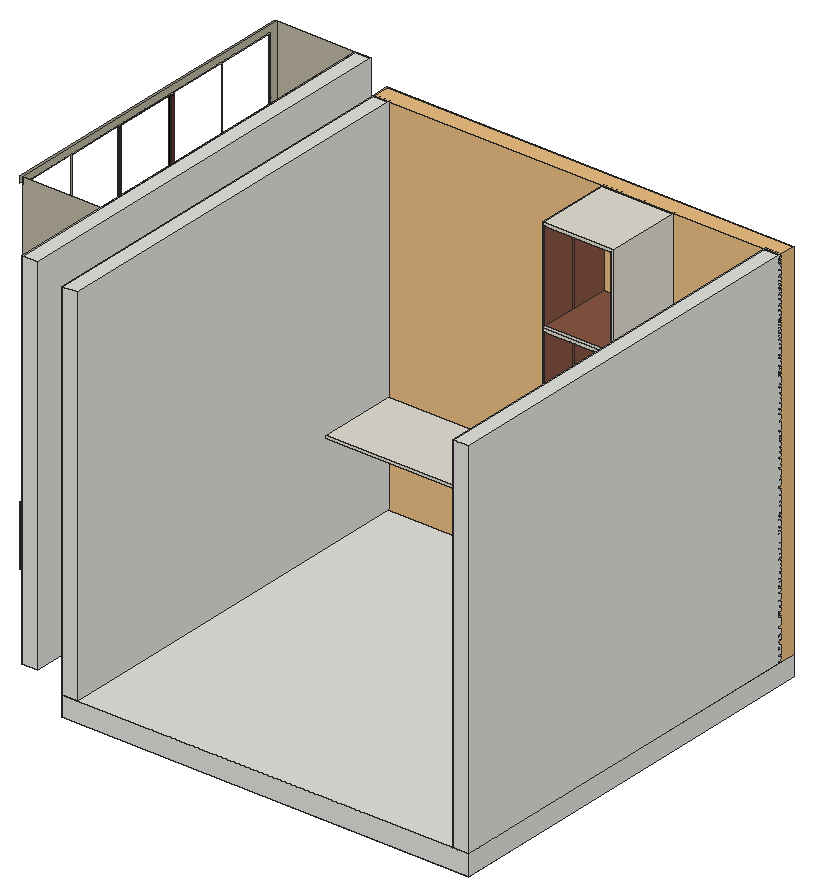
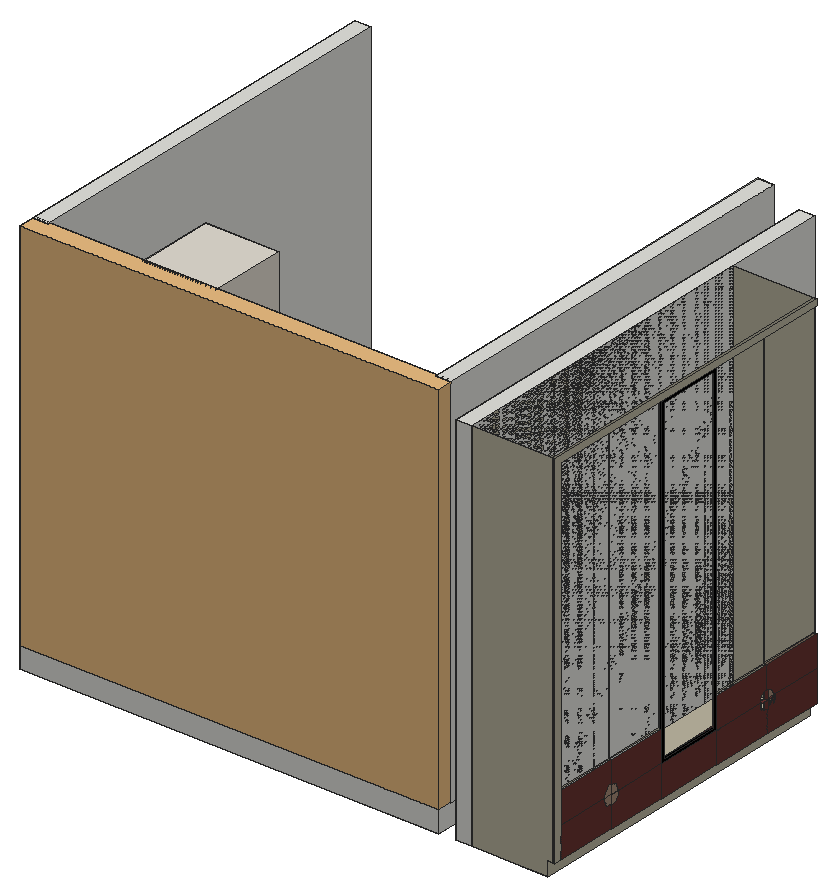
# SketchUp Ruby script. Lengths in millimetres.
U = 1.mm
M = Sketchup.active_model
def pt(a) = Geom::Point3d.new(a.map { |v| v * U })
def face(e, loops, mat)
  f = e.add_face(loops[0].map { |a| pt(a) })
  loops[1..].each { |l| e.add_face(l.map { |a| pt(a) }).erase! }
  f.material = f.back_material = mat if mat
  f
end
# faces: each face lists its corners as indices into pts; further lists are holes
def faces(e, pts, list, mat = nil) = list.each { |f| face(e, (f[0].is_a?(Array) ? f : [f]).map { |l| l.map { |i| pts[i] } }, mat) }
# xy, xz, yz: faces in a plane at the given z, y or x. An outline is a flat list of corners, or four numbers for a rectangle; further outlines are holes
def ring(l) = l.size == 4 ? [[l[0], l[1]], [l[2], l[1]], [l[2], l[3]], [l[0], l[3]]] : l.each_slice(2).to_a
def flat(e, list, mat, &to3) = list.each { |f| face(e, (f[0].is_a?(Array) ? f : [f]).map { |l| ring(l).map { |u, v| to3.(u, v) } }, mat) }
def xy(e, z, list, mat = nil) = flat(e, list, mat) { |x, y| [x, y, z] }
def xz(e, y, list, mat = nil) = flat(e, list, mat) { |x, z| [x, y, z] }
def yz(e, x, list, mat = nil) = flat(e, list, mat) { |y, z| [x, y, z] }
def lines(e, pts, list) = list.each { |a, b| e.add_line(pt(pts[a]), pt(pts[b])) }
# prism: a flat outline (further loops are holes) pulled along v
def prism(e, loops, v, mat = nil)
  f = face(e, loops, mat); d = Geom::Vector3d.new(v.map { |x| x * U })
  f.pushpull(f.normal.samedirection?(d) ? d.length : -d.length)
end
def box(e, o, s, mat = nil) = prism(e, [[o, [o[0] + s[0], o[1], o[2]], [o[0] + s[0], o[1] + s[1], o[2]], [o[0], o[1] + s[1], o[2]]]], [0, 0, s[2]], mat)
def at(x, y, z, deg = 0) = Geom::Transformation.translation(pt([x, y, z])) * Geom::Transformation.rotation(ORIGIN, Z_AXIS, deg.degrees)
def axes(o, x, y, z) = Geom::Transformation.new([*x, 0, *y, 0, *z, 0, *pt(o).to_a, 1])
def part(name) = M.definitions.add(name)
# library, detail: a bought-in or finely detailed component or shape, given as its bounding box
def library(name, o, s) = part(name).tap { |d| box(d.entities, o, s) }
def detail(e, o, s) = box(e.add_group.entities, o, s)
def put(e, d, t, mat = nil) = e.add_instance(d, t).tap { |i| i.material = mat if mat }
def group(e, t, mat = nil) = e.add_group.tap { |g| g.transformation = t; g.material = mat if mat }.entities
root = M.entities
M.materials.add("Olon-Fresh-Linen-VT10-1K").color = [226, 220, 209]
M.materials.add("Pionite-a-Panolam-Brand-Canyon-Shadow-SO200-4K").color = [135, 86, 67]
M.materials.add("Tafisa-Chateau-de-Sable-or-Sand-Castle-PM782-2K").color = [163, 138, 119]
M.materials.add("Uniboard-L17-Ambrette-4K").color = [104, 52, 49]
M.materials.add("Uniboard-L19-Putty-4K").color = [187, 181, 160]
M.materials.add("[Color M09]").color = [0, 0, 0]
c1 = library("Group\#21",[0,-18,0],[3048,132.3,2743.2])
c2 = part("Group282\#1")
p = [[0,0,0],[0,0,-404.7],[-1.4,0,-404.7],[9,-1301.3,0],[-9,-1301.3,0],[9,1301.3,0],
  [9,0,0],[-9,1301.3,0],[1.4,0,-404.7],[-9,0,0],[0,0,-655.2]]
lines(c2.entities,p,[[0,1],[1,2],[3,4],[5,6],[7,5],[1,8],[9,0],[0,6],[8,10],[4,9],[6,3],[2,10],
  [9,7]])
c3 = part("Rectangle Light\#2")
put(c3.entities,c2,at(0,0,0))
c4 = library("Group\#30",[0,0,0],[533.4,18,720.8])
c5 = part("Group280\#1")
p = [[0,0,0],[0,0,-404.7],[-1.4,0,-404.7],[9,-1301.3,0],[-9,-1301.3,0],[9,1301.3,0],
  [9,0,0],[-9,1301.3,0],[1.4,0,-404.7],[-9,0,0],[0,0,-655.2]]
lines(c5.entities,p,[[0,1],[1,2],[3,4],[5,6],[7,5],[1,8],[9,0],[0,6],[8,10],[4,9],[6,3],[2,10],
  [9,7]])
c6 = part("Rectangle Light\#1")
put(c6.entities,c5,at(0,0,0))
xy(root,152.4,[[2679.7,879.2,3238.5,3258.8]],"Uniboard-L19-Putty-4K")
xy(root,254,[[2628.9,879.2,2646.9,1333.4]],"Tafisa-Chateau-de-Sable-or-Sand-Castle-PM782-2K")
xy(root,254,[[2646.9,879.2,2646.9,1336.4,2628.9,1336.4,2628.9,1790.6,2646.9,1790.6,2646.9,1793.6,2628.9,1793.6,2628.9,2290.6,2646.9,2290.6,2646.9,2293.6,2628.9,2293.6,2628.9,2747.8,2646.9,2747.8,2646.9,2750.8,2628.9,2750.8,2628.9,3205,2646.9,3205,2646.9,3208,2679.7,3208,2679.7,879.2]],"Uniboard-L17-Ambrette-4K")
xy(root,254,[[2628.9,3208,2646.9,3258.8],[2646.9,3208,2679.7,3258.8]],"Uniboard-L19-Putty-4K")
xy(root,413.1,[[2628.9,1332.9,2646.9,1333.4]],"Tafisa-Chateau-de-Sable-or-Sand-Castle-PM782-2K")
xy(root,478.1,[[2628.9,879.2,2646.9,1269.9],[2619.9,1269.9,2646.9,1333.4],[2619.9,1336.4,2646.9,1336.4,2646.9,1790.6,2628.9,1790.6,2628.9,1399.9,2619.9,1399.9],[2628.9,1793.6,2646.9,2290.6],[2628.9,2293.6,2646.9,2747.8],
  [2628.9,2750.8,2646.9,3205]],"Uniboard-L17-Ambrette-4K")
xy(root,481.1,[[2628.9,879.2,2646.9,1269.9],[2619.9,1269.9,2631.9,1333.4],[2631.9,1269.9,2646.9,1333.4],[2619.9,1336.4,2619.9,1399.9,2628.9,1399.9,2628.9,1790.6,2646.9,1790.6,2646.9,1336.4],[2628.9,2293.6,2646.9,2747.8],
  [2628.9,2750.8,2646.9,3205]],"Uniboard-L17-Ambrette-4K")
xy(root,481.1,[[2628.9,1793.6,2646.9,2290.6],[2646.9,1793.6,2649.9,2290.6]],"Uniboard-L19-Putty-4K")
xz(root,879.2,[[2628.9,254,2646.9,478.1],[2628.9,481.1,2646.9,705.2]],"Uniboard-L17-Ambrette-4K")
xz(root,879.2,[[2679.7,152.4,3238.5,152.4,3238.5,2895.6,2646.9,2895.6,2646.9,254,2679.7,254]],"Uniboard-L19-Putty-4K")
xz(root,1269.9,[[2628.9,476.1,2646.9,478.1],[2628.9,481.1,2631.9,483.1],[2631.9,481.1,2646.9,483.1]],"Tafisa-Chateau-de-Sable-or-Sand-Castle-PM782-2K")
xz(root,1269.9,[[2619.9,476.1,2628.9,478.1],[2619.9,481.1,2628.9,483.1]],"Uniboard-L17-Ambrette-4K")
xz(root,1333.4,[[2628.9,254,2646.9,413.1],[2619.9,413.1,2646.9,478.1],[2619.9,481.1,2631.9,546.1],[2631.9,481.1,2646.9,546.1]],"Uniboard-L17-Ambrette-4K")
xz(root,1336.4,[[2628.9,254,2646.9,254,2646.9,478.1,2619.9,478.1,2619.9,413.1,2628.9,413.1],[2619.9,481.1,2646.9,481.1,2646.9,705.2,2628.9,705.2,2628.9,546.1,2619.9,546.1]],"Uniboard-L17-Ambrette-4K")
xz(root,1399.9,[[2619.9,476.1,2628.9,478.1],[2619.9,481.1,2628.9,483.1]],"Uniboard-L17-Ambrette-4K")
xz(root,1790.6,[[2628.9,254,2646.9,478.1],[2628.9,481.1,2646.9,705.2]],"Uniboard-L17-Ambrette-4K")
xz(root,1793.6,[[2628.9,254,2646.9,478.1]],"Uniboard-L17-Ambrette-4K")
xz(root,1793.6,[[2646.9,481.1,2649.9,2841.8]],"Uniboard-L19-Putty-4K")
xz(root,1793.6,[[2628.9,481.1,2646.9,2841.8]],"[Color M09]")
xz(root,2290.6,[[2628.9,254,2646.9,478.1]],"Uniboard-L17-Ambrette-4K")
xz(root,2290.6,[[2646.9,481.1,2649.9,2841.8]],"Uniboard-L19-Putty-4K")
xz(root,2290.6,[[2628.9,481.1,2646.9,2841.8]],"[Color M09]")
xz(root,2293.6,[[2628.9,254,2646.9,478.1],[2628.9,481.1,2646.9,705.2]],"Uniboard-L17-Ambrette-4K")
xz(root,2747.8,[[2628.9,254,2646.9,478.1],[2628.9,481.1,2646.9,705.2]],"Uniboard-L17-Ambrette-4K")
xz(root,2750.8,[[2628.9,254,2646.9,478.1],[2628.9,481.1,2646.9,705.2]],"Uniboard-L17-Ambrette-4K")
xz(root,3205,[[2628.9,254,2646.9,478.1]],"Tafisa-Chateau-de-Sable-or-Sand-Castle-PM782-2K")
xz(root,3205,[[2628.9,481.1,2646.9,705.2]],"Uniboard-L17-Ambrette-4K")
xz(root,3208,[[2628.9,254,2646.9,2844.8]],"Uniboard-L19-Putty-4K")
xz(root,3258.8,[[2679.7,152.4,2679.7,254,2646.9,254,2646.9,2895.6,3238.5,2895.6,3238.5,152.4],[2628.9,254,2646.9,2895.6]],"Uniboard-L19-Putty-4K")
yz(root,2628.9,[[2747.3,413.1,2747.8,413.1,2747.8,478.1,2684.3,478.1,2684.3,476.1,2684.4,474,2684.8,470,2685.1,467.9,2686.3,461.9,2686.9,460,2687.5,458,2688.1,456.1,2690.5,450.4,2692.3,446.8,2693.4,445,2694.4,443.3,2695.5,441.6,2696.7,439.9,2697.9,438.3,2700.5,435.1,2703.3,432.1,2706.3,429.3,2709.5,426.7,2711.1,425.5,2712.8,424.3,2714.5,423.2,2716.2,422.2,2718,421.1,2721.6,419.3,2723.5,418.4,2725.4,417.7,2727.3,416.9,2729.2,416.3,2731.2,415.7,2733.1,415.1,2739.1,413.9,2741.2,413.6,2745.2,413.2],[2750.8,413.1,2751.3,413.1,2753.4,413.2,2755.4,413.4,2757.5,413.6,2759.5,413.9,2765.5,415.1,2767.4,415.7,2769.4,416.3,2771.3,416.9,2773.2,417.7,2775.1,418.4,2777,419.3,2780.6,421.1,2782.4,422.2,2784.1,423.2,2785.8,424.3,2787.5,425.5,2789.1,426.7,2792.3,429.3,2795.3,432.1,2798.1,435.1,2800.7,438.3,2801.9,439.9,2803.1,441.6,2805.3,445,2806.3,446.8,2808.1,450.4,2809,452.3,2809.7,454.2,2810.5,456.1,2811.1,458,2811.7,460,2812.3,461.9,2812.7,463.9,2813.2,465.9,2813.5,467.9,2813.8,470,2814.2,474,2814.3,476.1,2814.3,478.1,2750.8,478.1],[2684.3,481.1,2747.8,481.1,2747.8,546.1,2747.3,546.1,2745.2,546,2741.2,545.6,2739.1,545.3,2733.1,544.1,2731.2,543.5,2729.2,542.9,2727.3,542.3,2725.4,541.5,2723.5,540.8,2721.6,539.9,2718,538.1,2716.2,537,2714.5,536,2712.8,534.9,2711.1,533.7,2709.5,532.5,2706.3,529.9,2703.3,527.1,2700.5,524.1,2697.9,520.9,2696.7,519.3,2695.5,517.6,2694.4,515.9,2693.4,514.2,2692.3,512.4,2690.5,508.8,2688.1,503.1,2687.5,501.2,2686.9,499.2,2686.3,497.3,2685.1,491.3,2684.8,489.2,2684.4,485.2,2684.3,483.1],[2750.8,481.1,2814.3,481.1,2814.3,483.1,2814.2,485.2,2813.8,489.2,2813.5,491.3,2813.2,493.3,2812.7,495.3,2812.3,497.3,2811.7,499.2,2811.1,501.2,2810.5,503.1,2809.7,505,2809,506.9,2808.1,508.8,2806.3,512.4,2805.3,514.2,2803.1,517.6,2801.9,519.3,2800.7,520.9,2798.1,524.1,2795.3,527.1,2792.3,529.9,2789.1,532.5,2787.5,533.7,2785.8,534.9,2784.1,536,2782.4,537,2780.6,538.1,2777,539.9,2775.1,540.8,2773.2,541.5,2771.3,542.3,2769.4,542.9,2767.4,543.5,2765.5,544.1,2759.5,545.3,2757.5,545.6,2755.4,545.8,2753.4,546,2751.3,546.1,2750.8,546.1]],"Tafisa-Chateau-de-Sable-or-Sand-Castle-PM782-2K")
yz(root,2628.9,[[879.2,254,879.2,478.1,1269.9,478.1,1269.9,476.1,1270,474,1270.4,470,1270.7,467.9,1271.9,461.9,1272.5,460,1273.1,458,1273.7,456.1,1276.1,450.4,1277.9,446.8,1279,445,1280,443.3,1281.1,441.6,1282.3,439.9,1283.5,438.3,1286.1,435.1,1288.9,432.1,1291.9,429.3,1295.1,426.7,1296.7,425.5,1298.4,424.3,1300.1,423.2,1301.8,422.2,1303.6,421.1,1307.2,419.3,1309.1,418.4,1311,417.7,1312.9,416.9,1314.8,416.3,1316.8,415.7,1318.7,415.1,1324.7,413.9,1326.8,413.6,1330.8,413.2,1332.9,413.1,1333.4,413.1,1333.4,254],[1336.4,254,1336.4,413.1,1336.9,413.1,1339,413.2,1341,413.4,1343.1,413.6,1345.1,413.9,1351.1,415.1,1353,415.7,1355,416.3,1356.9,416.9,1358.8,417.7,1360.7,418.4,1362.6,419.3,1366.2,421.1,1368,422.2,1369.7,423.2,1371.4,424.3,1373.1,425.5,1374.7,426.7,1377.9,429.3,1380.9,432.1,1383.7,435.1,1386.3,438.3,1387.5,439.9,1388.7,441.6,1390.9,445,1391.9,446.8,1393.7,450.4,1394.6,452.3,1395.3,454.2,1396.1,456.1,1396.7,458,1397.3,460,1397.9,461.9,1398.3,463.9,1398.8,465.9,1399.1,467.9,1399.4,470,1399.8,474,1399.9,476.1,1399.9,478.1,1790.6,478.1,1790.6,254],[1793.6,254,2290.6,478.1],[2293.6,254,2293.6,478.1,2684.3,478.1,2684.3,476.1,2684.4,474,2684.8,470,2685.1,467.9,2686.3,461.9,2686.9,460,2687.5,458,2688.1,456.1,2690.5,450.4,2692.3,446.8,2693.4,445,2694.4,443.3,2695.5,441.6,2696.7,439.9,2697.9,438.3,2700.5,435.1,2703.3,432.1,2706.3,429.3,2709.5,426.7,2711.1,425.5,2712.8,424.3,2714.5,423.2,2716.2,422.2,2718,421.1,2721.6,419.3,2723.5,418.4,2725.4,417.7,2727.3,416.9,2729.2,416.3,2731.2,415.7,2733.1,415.1,2739.1,413.9,2741.2,413.6,2745.2,413.2,2747.3,413.1,2747.8,413.1,2747.8,254],[2750.8,254,2750.8,413.1,2751.3,413.1,2753.4,413.2,2755.4,413.4,2757.5,413.6,2759.5,413.9,2765.5,415.1,2767.4,415.7,2769.4,416.3,2771.3,416.9,2773.2,417.7,2775.1,418.4,2777,419.3,2780.6,421.1,2782.4,422.2,2784.1,423.2,2785.8,424.3,2787.5,425.5,2789.1,426.7,2792.3,429.3,2795.3,432.1,2798.1,435.1,2800.7,438.3,2801.9,439.9,2803.1,441.6,2805.3,445,2806.3,446.8,2808.1,450.4,2809,452.3,2809.7,454.2,2810.5,456.1,2811.1,458,2811.7,460,2812.3,461.9,2812.7,463.9,2813.2,465.9,2813.5,467.9,2813.8,470,2814.2,474,2814.3,476.1,2814.3,478.1,3205,478.1,3205,254],
  [879.2,481.1,879.2,705.2,1333.4,705.2,1333.4,546.1,1332.9,546.1,1330.8,546,1326.8,545.6,1324.7,545.3,1318.7,544.1,1316.8,543.5,1314.8,542.9,1312.9,542.3,1311,541.5,1309.1,540.8,1307.2,539.9,1303.6,538.1,1301.8,537,1300.1,536,1298.4,534.9,1296.7,533.7,1295.1,532.5,1291.9,529.9,1288.9,527.1,1286.1,524.1,1283.5,520.9,1282.3,519.3,1281.1,517.6,1280,515.9,1279,514.2,1277.9,512.4,1276.1,508.8,1273.7,503.1,1273.1,501.2,1272.5,499.2,1271.9,497.3,1270.7,491.3,1270.4,489.2,1270,485.2,1269.9,483.1,1269.9,481.1],[1399.9,481.1,1399.9,483.1,1399.8,485.2,1399.4,489.2,1399.1,491.3,1398.8,493.3,1398.3,495.3,1397.9,497.3,1397.3,499.2,1396.7,501.2,1396.1,503.1,1395.3,505,1394.6,506.9,1393.7,508.8,1391.9,512.4,1390.9,514.2,1388.7,517.6,1387.5,519.3,1386.3,520.9,1383.7,524.1,1380.9,527.1,1377.9,529.9,1374.7,532.5,1373.1,533.7,1371.4,534.9,1369.7,536,1368,537,1366.2,538.1,1362.6,539.9,1360.7,540.8,1358.8,541.5,1356.9,542.3,1355,542.9,1353,543.5,1351.1,544.1,1345.1,545.3,1343.1,545.6,1341,545.8,1339,546,1336.9,546.1,1336.4,546.1,1336.4,705.2,1790.6,705.2,1790.6,481.1],[2293.6,481.1,2293.6,705.2,2747.8,705.2,2747.8,546.1,2747.3,546.1,2745.2,546,2741.2,545.6,2739.1,545.3,2733.1,544.1,2731.2,543.5,2729.2,542.9,2727.3,542.3,2725.4,541.5,2723.5,540.8,2721.6,539.9,2718,538.1,2716.2,537,2714.5,536,2712.8,534.9,2711.1,533.7,2709.5,532.5,2706.3,529.9,2703.3,527.1,2700.5,524.1,2697.9,520.9,2696.7,519.3,2695.5,517.6,2694.4,515.9,2693.4,514.2,2692.3,512.4,2690.5,508.8,2688.1,503.1,2687.5,501.2,2686.9,499.2,2686.3,497.3,2685.1,491.3,2684.8,489.2,2684.4,485.2,2684.3,483.1,2684.3,481.1],[2814.3,481.1,2814.3,483.1,2814.2,485.2,2813.8,489.2,2813.5,491.3,2813.2,493.3,2812.7,495.3,2812.3,497.3,2811.7,499.2,2811.1,501.2,2810.5,503.1,2809.7,505,2809,506.9,2808.1,508.8,2806.3,512.4,2805.3,514.2,2803.1,517.6,2801.9,519.3,2800.7,520.9,2798.1,524.1,2795.3,527.1,2792.3,529.9,2789.1,532.5,2787.5,533.7,2785.8,534.9,2784.1,536,2782.4,537,2780.6,538.1,2777,539.9,2775.1,540.8,2773.2,541.5,2771.3,542.3,2769.4,542.9,2767.4,543.5,2765.5,544.1,2759.5,545.3,2757.5,545.6,2755.4,545.8,2753.4,546,2751.3,546.1,2750.8,546.1,2750.8,705.2,3205,705.2,3205,481.1]],"Uniboard-L17-Ambrette-4K")
yz(root,2628.9,[[3208,254,3208,2844.8,879.2,2844.8,879.2,2895.6,3258.8,2895.6,3258.8,254]],"Uniboard-L19-Putty-4K")
yz(root,2628.9,[[[1793.6,481.1,2290.6,2841.8],[1811.6,499.1,2272.6,2823.8]]],"[Color M09]")
yz(root,2631.9,[[1269.9,481.1,1333.4,481.1,1333.4,546.1,1332.9,546.1,1330.8,546,1326.8,545.6,1324.7,545.3,1318.7,544.1,1316.8,543.5,1314.8,542.9,1312.9,542.3,1311,541.5,1309.1,540.8,1307.2,539.9,1303.6,538.1,1301.8,537,1300.1,536,1298.4,534.9,1296.7,533.7,1295.1,532.5,1291.9,529.9,1288.9,527.1,1286.1,524.1,1283.5,520.9,1282.3,519.3,1281.1,517.6,1280,515.9,1279,514.2,1277.9,512.4,1276.1,508.8,1273.7,503.1,1273.1,501.2,1272.5,499.2,1271.9,497.3,1270.7,491.3,1270.4,489.2,1270,485.2,1269.9,483.1]],"Tafisa-Chateau-de-Sable-or-Sand-Castle-PM782-2K")
yz(root,2646.9,[[879.2,254,1333.4,254,1333.4,413.1,1332.9,413.1,1330.8,413.2,1326.8,413.6,1324.7,413.9,1318.7,415.1,1316.8,415.7,1314.8,416.3,1312.9,416.9,1311,417.7,1309.1,418.4,1307.2,419.3,1303.6,421.1,1301.8,422.2,1300.1,423.2,1298.4,424.3,1296.7,425.5,1295.1,426.7,1291.9,429.3,1288.9,432.1,1286.1,435.1,1283.5,438.3,1282.3,439.9,1281.1,441.6,1280,443.3,1279,445,1277.9,446.8,1276.1,450.4,1273.7,456.1,1273.1,458,1272.5,460,1271.9,461.9,1270.7,467.9,1270.4,470,1270,474,1269.9,476.1,1269.9,478.1,879.2,478.1],[879.2,481.1,1269.9,481.1,1269.9,483.1,1270,485.2,1270.4,489.2,1270.7,491.3,1271.9,497.3,1272.5,499.2,1273.1,501.2,1273.7,503.1,1276.1,508.8,1277.9,512.4,1279,514.2,1280,515.9,1281.1,517.6,1282.3,519.3,1283.5,520.9,1286.1,524.1,1288.9,527.1,1291.9,529.9,1295.1,532.5,1296.7,533.7,1298.4,534.9,1300.1,536,1301.8,537,1303.6,538.1,1307.2,539.9,1309.1,540.8,1311,541.5,1312.9,542.3,1314.8,542.9,1316.8,543.5,1318.7,544.1,1324.7,545.3,1326.8,545.6,1330.8,546,1332.9,546.1,1333.4,546.1,1333.4,705.2,879.2,705.2]],"Tafisa-Chateau-de-Sable-or-Sand-Castle-PM782-2K")
yz(root,2646.9,[[3208,254,3258.8,254,3258.8,2895.6,879.2,2895.6,879.2,2844.8,3208,2844.8],[[1333.4,254,1333.4,478.1,879.2,478.1,879.2,481.1,1333.4,481.1,1333.4,705.2,879.2,705.2,879.2,708.2,1333.4,708.2,1333.4,2841.8,879.2,2841.8,879.2,2844.8,3208,2844.8,3208,254,3205,254,3205,478.1,2750.8,478.1,2750.8,254,2747.8,254,2747.8,478.1,2293.6,478.1,2293.6,254,2290.6,254,2290.6,478.1,1793.6,478.1,1793.6,254,1790.6,254,1790.6,478.1,1336.4,478.1,1336.4,254],[1793.6,481.1,2290.6,2841.8],[2293.6,708.2,2747.8,2841.8],[2750.8,708.2,3205,2841.8],[1336.4,708.2,1790.6,2841.8],[2293.6,481.1,2747.8,705.2],[2750.8,481.1,3205,705.2],[1336.4,481.1,1790.6,705.2]]],"Uniboard-L19-Putty-4K")
yz(root,2646.9,[[1793.6,481.1,2272.6,499.1],[2272.6,481.1,2290.6,2823.8]],"[Color M09]")
yz(root,2649.9,[[1793.6,481.1,1793.6,499.1,2272.6,499.1,2272.6,2823.8,2290.6,2823.8,2290.6,481.1]],"Uniboard-L17-Ambrette-4K")
yz(root,2679.7,[[879.2,152.4,3258.8,254]],"Uniboard-L19-Putty-4K")
yz(root,3238.5,[[879.2,152.4,3258.8,2895.6]],"Uniboard-L19-Putty-4K")
p = [[2628.9,1332.9,413.1],[2628.9,1330.8,413.2],[2646.9,1330.8,413.2],[2646.9,1332.9,413.1],[2628.9,1328.8,413.4],[2646.9,1328.8,413.4],
  [2628.9,1326.8,413.6],[2646.9,1326.8,413.6],[2628.9,1324.7,413.9],[2646.9,1324.7,413.9],[2628.9,1322.7,414.3],[2646.9,1322.7,414.3],
  [2628.9,1320.7,414.7],[2646.9,1320.7,414.7],[2628.9,1318.7,415.1],[2646.9,1318.7,415.1],[2628.9,1316.8,415.7],[2646.9,1316.8,415.7],
  [2628.9,1314.8,416.3],[2646.9,1314.8,416.3],[2628.9,1312.9,416.9],[2646.9,1312.9,416.9],[2628.9,1311,417.7],[2646.9,1311,417.7],
  [2628.9,1309.1,418.4],[2646.9,1309.1,418.4],[2628.9,1307.2,419.3],[2646.9,1307.2,419.3],[2628.9,1305.4,420.2],[2646.9,1305.4,420.2],
  [2628.9,1303.6,421.1],[2646.9,1303.6,421.1],[2628.9,1301.8,422.2],[2646.9,1301.8,422.2],[2628.9,1300.1,423.2],[2646.9,1300.1,423.2],
  [2628.9,1298.4,424.3],[2646.9,1298.4,424.3],[2628.9,1296.7,425.5],[2646.9,1296.7,425.5],[2628.9,1295.1,426.7],[2646.9,1295.1,426.7],
  [2628.9,1293.5,428],[2646.9,1293.5,428],[2628.9,1291.9,429.3],[2646.9,1291.9,429.3],[2628.9,1290.4,430.7],[2646.9,1290.4,430.7],
  [2628.9,1288.9,432.1],[2646.9,1288.9,432.1],[2628.9,1287.5,433.6],[2646.9,1287.5,433.6],[2628.9,1286.1,435.1],[2646.9,1286.1,435.1],
  [2628.9,1284.8,436.7],[2646.9,1284.8,436.7],[2628.9,1283.5,438.3],[2646.9,1283.5,438.3],[2628.9,1282.3,439.9],[2619.9,1282.3,439.9],
  [2619.9,1283.5,438.3],[2646.9,1282.3,439.9],[2628.9,1387.5,439.9],[2628.9,1386.3,438.3],[2619.9,1386.3,438.3],[2619.9,1387.5,439.9],
  [2628.9,1281.1,441.6],[2619.9,1281.1,441.6],[2646.9,1281.1,441.6],[2628.9,1388.7,441.6],[2619.9,1388.7,441.6],[2628.9,1280,443.3],
  [2619.9,1280,443.3],[2646.9,1280,443.3],[2628.9,1389.8,443.3],[2619.9,1389.8,443.3],[2628.9,1279,445],[2619.9,1279,445],
  [2646.9,1279,445],[2628.9,1390.9,445],[2619.9,1390.9,445],[2628.9,1277.9,446.8],[2619.9,1277.9,446.8],[2646.9,1277.9,446.8],
  [2628.9,1391.9,446.8],[2619.9,1391.9,446.8],[2628.9,1277,448.6],[2619.9,1277,448.6],[2646.9,1277,448.6],[2628.9,1392.8,448.6],
  [2619.9,1392.8,448.6],[2628.9,1276.1,450.4],[2619.9,1276.1,450.4],[2646.9,1276.1,450.4],[2628.9,1393.7,450.4],[2619.9,1393.7,450.4],
  [2628.9,1275.3,452.3],[2619.9,1275.3,452.3],[2646.9,1275.3,452.3],[2628.9,1394.6,452.3],[2619.9,1394.6,452.3],[2628.9,1274.5,454.2],
  [2619.9,1274.5,454.2],[2646.9,1274.5,454.2],[2628.9,1395.3,454.2],[2619.9,1395.3,454.2],[2628.9,1273.7,456.1],[2619.9,1273.7,456.1],
  [2646.9,1273.7,456.1],[2628.9,1396.1,456.1],[2619.9,1396.1,456.1],[2628.9,1273.1,458],[2619.9,1273.1,458],[2646.9,1273.1,458],
  [2628.9,1396.7,458],[2619.9,1396.7,458],[2628.9,1272.5,460],[2619.9,1272.5,460],[2646.9,1272.5,460],[2628.9,1397.3,460],
  [2619.9,1397.3,460],[2628.9,1271.9,461.9],[2619.9,1271.9,461.9],[2646.9,1271.9,461.9],[2628.9,1397.9,461.9],[2619.9,1397.9,461.9],
  [2628.9,1271.5,463.9],[2619.9,1271.5,463.9],[2646.9,1271.5,463.9],[2628.9,1398.3,463.9],[2619.9,1398.3,463.9],[2628.9,1271.1,465.9],
  [2619.9,1271.1,465.9],[2646.9,1271.1,465.9],[2628.9,1398.8,465.9],[2619.9,1398.8,465.9],[2628.9,1270.7,467.9],[2619.9,1270.7,467.9],
  [2646.9,1270.7,467.9],[2628.9,1399.1,467.9],[2619.9,1399.1,467.9],[2628.9,1270.4,470],[2619.9,1270.4,470],[2646.9,1270.4,470],
  [2628.9,1399.4,470],[2619.9,1399.4,470],[2628.9,1270.2,472],[2619.9,1270.2,472],[2646.9,1270.2,472],[2628.9,1399.6,472],
  [2619.9,1399.6,472],[2628.9,1270,474],[2619.9,1270,474],[2646.9,1270,474],[2628.9,1399.8,474],[2619.9,1399.8,474],
  [2628.9,1269.9,476.1],[2619.9,1269.9,476.1],[2646.9,1269.9,476.1],[2628.9,1399.9,476.1],[2619.9,1399.9,476.1],[2628.9,1269.9,483.1],
  [2628.9,1270,485.2],[2619.9,1270,485.2],[2619.9,1269.9,483.1],[2631.9,1270,485.2],[2631.9,1269.9,483.1],[2646.9,1269.9,483.1],
  [2646.9,1270,485.2],[2628.9,1399.8,485.2],[2628.9,1399.9,483.1],[2619.9,1399.9,483.1],[2619.9,1399.8,485.2],[2628.9,1270.2,487.2],
  [2619.9,1270.2,487.2],[2631.9,1270.2,487.2],[2646.9,1270.2,487.2],[2628.9,1399.6,487.2],[2619.9,1399.6,487.2],[2628.9,1270.4,489.2],
  [2619.9,1270.4,489.2],[2631.9,1270.4,489.2],[2628.9,1399.4,489.2],[2619.9,1399.4,489.2],[2628.9,2749.3,413.1],[2628.9,2747.8,413.1],
  [2628.9,2750.8,413.1],[2628.9,1334.9,413.1],[2628.9,1333.4,413.1],[2628.9,1336.4,413.1]]
faces(root,p,[[0,1,2,3],[1,4,5,2],[4,6,7,5],[6,8,9,7],[8,10,11,9],[10,12,13,11],[12,14,15,13],[14,16,17,15],
  [16,18,19,17],[18,20,21,19],[20,22,23,21],[22,24,25,23],[24,26,27,25],[26,28,29,27],[28,30,31,29],[30,32,33,31],
  [32,34,35,33],[34,36,37,35],[36,38,39,37],[38,40,41,39],[40,42,43,41],[42,44,45,43],[44,46,47,45],[46,48,49,47],
  [48,50,51,49],[50,52,53,51],[52,54,55,53],[54,56,57,55],[56,58,61,57],[58,66,68,61],[66,71,73,68],[71,76,78,73],
  [76,81,83,78],[81,86,88,83],[86,91,93,88],[91,96,98,93],[96,101,103,98],[101,106,108,103],[106,111,113,108],[111,116,118,113],
  [116,121,123,118],[121,126,128,123],[126,131,133,128],[131,136,138,133],[136,141,143,138],[141,146,148,143],[146,151,153,148],[151,156,158,153],
  [162,165,166,161],[167,166,165,168],[173,175,165,162],[168,165,175,176],[179,181,175,173]],"Tafisa-Chateau-de-Sable-or-Sand-Castle-PM782-2K")
faces(root,p,[[56,58,59,60],[62,63,64,65],[58,66,67,59],[69,62,65,70],[66,71,72,67],[74,69,70,75],[71,76,77,72],[79,74,75,80],
  [76,81,82,77],[84,79,80,85],[81,86,87,82],[89,84,85,90],[86,91,92,87],[94,89,90,95],[91,96,97,92],[99,94,95,100],
  [96,101,102,97],[104,99,100,105],[101,106,107,102],[109,104,105,110],[106,111,112,107],[114,109,110,115],[111,116,117,112],[119,114,115,120],
  [116,121,122,117],[124,119,120,125],[121,126,127,122],[129,124,125,130],[126,131,132,127],[134,129,130,135],[131,136,137,132],[139,134,135,140],
  [136,141,142,137],[144,139,140,145],[141,146,147,142],[149,144,145,150],[146,151,152,147],[154,149,150,155],[151,156,157,152],[159,154,155,160],
  [161,162,163,164],[169,170,171,172],[162,173,174,163],[177,169,172,178],[173,179,180,174],[182,177,178,183]],"Uniboard-L17-Ambrette-4K")
lines(root,p,[[184,185],[186,184],[187,188],[189,187]])
g1 = group(root,at(3238.5,134.6,152.4))
box(g1,[0,0,0],[114.3,3124.2,2743.2])
g2 = group(root,at(3761.6,2324.1,152.4),"Olon-Fresh-Linen-VT10-1K")
xy(g2,0,[[1066.8,50.8,2133.6,609.6]])
xy(g2,101.6,[[1066.8,0,1600.2,18],[1066.8,18,1600.2,50.8],[1600.2,36,2133.6,50.8]])
xy(g2,119.6,[[1618.2,36,2115.6,598]],"Pionite-a-Panolam-Brand-Canyon-Shadow-SO200-4K")
xy(g2,312.1,[[1066.8,0,1600.2,18]])
xy(g2,315.1,[[1066.8,0,1600.2,18]])
xy(g2,525.5,[[1066.8,0,1600.2,18]])
xy(g2,528.5,[[1066.8,0,1600.2,18]])
xy(g2,739,[[1066.8,0,1600.2,18]])
xy(g2,742,[[0,0,1066.8,609.6],[1066.8,0,1600.2,18]])
xy(g2,762,[[0,0,1600.2,609.6]])
xy(g2,805.9,[[1618.2,36,2115.6,598]],"Pionite-a-Panolam-Brand-Canyon-Shadow-SO200-4K")
xy(g2,841.9,[[1618.2,36,2115.6,598]],"Pionite-a-Panolam-Brand-Canyon-Shadow-SO200-4K")
xy(g2,2011,[[1618.2,36,2115.6,598]],"Pionite-a-Panolam-Brand-Canyon-Shadow-SO200-4K")
xy(g2,2047,[[1618.2,36,2115.6,598]],"Pionite-a-Panolam-Brand-Canyon-Shadow-SO200-4K")
xy(g2,2722.2,[[1618.2,36,2115.6,598]],"Pionite-a-Panolam-Brand-Canyon-Shadow-SO200-4K")
xy(g2,2740.2,[[1600.2,36,2133.6,609.6]])
xz(g2,0,[[1066.8,101.6,1600.2,312.1],[1066.8,315.1,1600.2,525.5],[1066.8,528.5,1600.2,739],[0,742,1600.2,762]])
xz(g2,18,[[1066.8,101.6,1600.2,312.1],[1066.8,312.1,1600.2,315.1],[1066.8,315.1,1600.2,525.5],[1066.8,525.5,1600.2,528.5],[1066.8,528.5,1600.2,739],
  [1066.8,739,1600.2,742]])
xz(g2,36,[[[1600.2,101.6,2133.6,823.9],[1618.2,119.6,2115.6,805.9]],[[1600.2,823.9,2133.6,2029],[1618.2,841.9,2115.6,2011]],[[1600.2,2029,2133.6,2740.2],[1618.2,2047,2115.6,2722.2]]])
xz(g2,50.8,[[1066.8,0,2133.6,101.6]])
xz(g2,598,[[1618.2,119.6,2115.6,805.9],[1618.2,841.9,2115.6,2011],[1618.2,2047,2115.6,2722.2]],"Pionite-a-Panolam-Brand-Canyon-Shadow-SO200-4K")
xz(g2,609.6,[[1066.8,0,1066.8,742,0,742,0,762,1600.2,762,1600.2,2740.2,2133.6,2740.2,2133.6,0]])
yz(g2,0,[[0,742,609.6,762]])
yz(g2,1066.8,[[50.8,0,50.8,101.6,18,101.6,18,742,609.6,742,609.6,0],[0,101.6,18,312.1],[0,315.1,18,525.5],[0,528.5,18,739]])
yz(g2,1600.2,[[0,101.6,18,312.1],[18,101.6,36,312.1],[18,312.1,36,315.1],[0,315.1,18,525.5],[18,315.1,36,525.5],
  [18,525.5,36,528.5],[0,528.5,18,739],[18,528.5,36,739],[18,739,36,742],[0,742,36,762],
  [36,762,609.6,2740.2]])
yz(g2,1618.2,[[36,119.6,598,739],[36,739,598,742],[36,742,598,762],[36,762,598,805.9],[36,841.9,598,2011],
  [36,2047,598,2722.2]],"Pionite-a-Panolam-Brand-Canyon-Shadow-SO200-4K")
yz(g2,2115.6,[[36,119.6,598,805.9],[36,841.9,598,2011],[36,2047,598,2722.2]],"Pionite-a-Panolam-Brand-Canyon-Shadow-SO200-4K")
yz(g2,2133.6,[[50.8,0,609.6,0,609.6,2740.2,36,2740.2,36,101.6,50.8,101.6]])
put(root,c1,at(3647.3,2933.7,152.4))
g3 = group(root,at(3647.3,0,0))
box(g3,[0,0,0],[3048,3048,152.4])
g4 = group(g3,at(2933.7,0,152.4))
box(g4,[0,0,0],[114.3,2933.7,2743.2])
g5 = group(g3,at(0,0,152.4))
box(g5,[0,0,0],[114.3,2933.7,2743.2])
put(root,c3,axes([5876.9,2632.1,1573.3],[0,-1,0],[0,0,1],[1,0,0]))
put(root,c4,at(5361.8,2342.1,254),"Olon-Fresh-Linen-VT10-1K")
put(root,c6,axes([5380,2632.1,1573.3],[0,-1,0],[0,0,1],[-1,0,0]))
